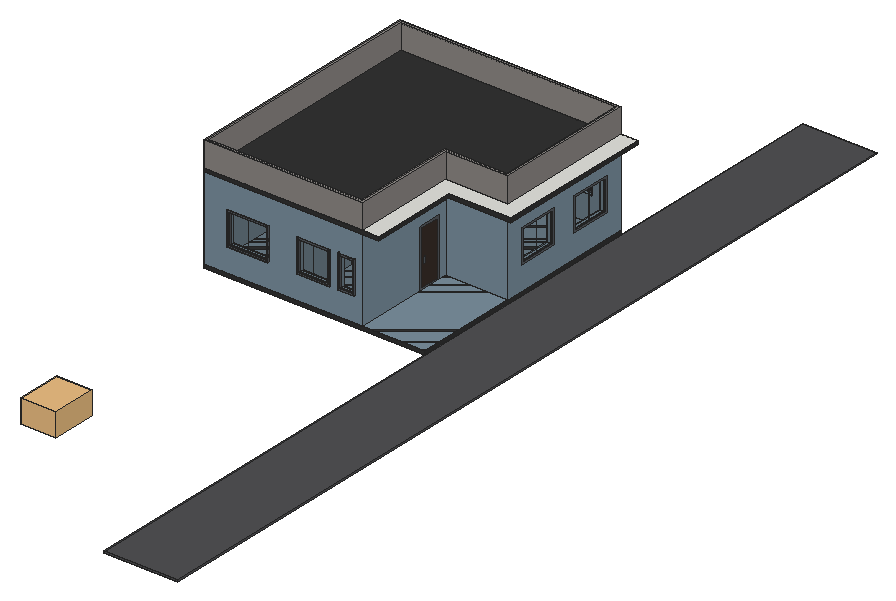
# SketchUp Ruby script. Lengths in inches.
U = 1.inch
M = Sketchup.active_model
def pt(a) = Geom::Point3d.new(a.map { |v| v * U })
def face(e, loops, mat)
  f = e.add_face(loops[0].map { |a| pt(a) })
  loops[1..].each { |l| e.add_face(l.map { |a| pt(a) }).erase! }
  f.material = f.back_material = mat if mat
  f
end
# faces: each face lists its corners as indices into pts; further lists are holes
def faces(e, pts, list, mat = nil) = list.each { |f| face(e, (f[0].is_a?(Array) ? f : [f]).map { |l| l.map { |i| pts[i] } }, mat) }
# xy, xz, yz: faces in a plane at the given z, y or x. An outline is a flat list of corners, or four numbers for a rectangle; further outlines are holes
def ring(l) = l.size == 4 ? [[l[0], l[1]], [l[2], l[1]], [l[2], l[3]], [l[0], l[3]]] : l.each_slice(2).to_a
def flat(e, list, mat, &to3) = list.each { |f| face(e, (f[0].is_a?(Array) ? f : [f]).map { |l| ring(l).map { |u, v| to3.(u, v) } }, mat) }
def xy(e, z, list, mat = nil) = flat(e, list, mat) { |x, y| [x, y, z] }
def xz(e, y, list, mat = nil) = flat(e, list, mat) { |x, z| [x, y, z] }
def yz(e, x, list, mat = nil) = flat(e, list, mat) { |y, z| [x, y, z] }
def lines(e, pts, list) = list.each { |a, b| e.add_line(pt(pts[a]), pt(pts[b])) }
# prism: a flat outline (further loops are holes) pulled along v
def prism(e, loops, v, mat = nil)
  f = face(e, loops, mat); d = Geom::Vector3d.new(v.map { |x| x * U })
  f.pushpull(f.normal.samedirection?(d) ? d.length : -d.length)
end
def box(e, o, s, mat = nil) = prism(e, [[o, [o[0] + s[0], o[1], o[2]], [o[0] + s[0], o[1] + s[1], o[2]], [o[0], o[1] + s[1], o[2]]]], [0, 0, s[2]], mat)
def at(x, y, z, deg = 0) = Geom::Transformation.translation(pt([x, y, z])) * Geom::Transformation.rotation(ORIGIN, Z_AXIS, deg.degrees)
def axes(o, x, y, z) = Geom::Transformation.new([*x, 0, *y, 0, *z, 0, *pt(o).to_a, 1])
def part(name) = M.definitions.add(name)
# library, detail: a bought-in or finely detailed component or shape, given as its bounding box
def library(name, o, s) = part(name).tap { |d| box(d.entities, o, s) }
def detail(e, o, s) = box(e.add_group.entities, o, s)
def put(e, d, t, mat = nil) = e.add_instance(d, t).tap { |i| i.material = mat if mat }
def group(e, t, mat = nil) = e.add_group.tap { |g| g.transformation = t; g.material = mat if mat }.entities
root = M.entities
M.materials.add("Asphalt A01 100cm").color = [81, 81, 83]
M.materials.add("Glass Smoked Distorted 001").color = [38, 38, 38]
M.materials["Glass Smoked Distorted 001"].alpha = 0.1
M.materials.add("Metal Sandblasted Black 200cm").color = [86, 90, 95]
M.materials.add("Two Color Maple Panels 300cm").color = [56, 46, 41]
M.materials.add("Venetian Plaster Black 300cm").color = [50, 50, 50]
M.materials.add("Wall Paint Dusk Blue Semigloss 300cm").color = [122, 143, 157]
M.materials.add("Wall Paint Poised Taupe Satin 300cm").color = [140, 135, 132]
c1 = library("Dome Light",[-12,-12,0],[24,24,12])
c2 = part("Group\#18")
box(c2.entities,[0,0,0],[28,0.31,44])
c3 = part("Group\#20")
box(c3.entities,[0,0,0],[22,0.31,44])
c4 = part("Group\#24")
box(c4.entities,[-0.31,0,0],[0.31,28,44])
c5 = part("Group\#26")
box(c5.entities,[-0.31,0,0],[0.31,28,44])
c6 = part("Group\#28")
box(c6.entities,[0,-0.31,0],[28,0.31,44])
c7 = part("Group\#30")
box(c7.entities,[0,-0.31,0],[28,0.31,44])
c8 = part("Group\#32")
box(c8.entities,[-0.31,0,0],[0.31,20,2])
c9 = part("Group\#34")
box(c9.entities,[-0.31,0,0],[0.31,20,2])
xy(root,137.15,[[234.81,586.875,258.81,586.875,258.81,714.875,349.81,714.875,349.81,946.875,325.81,946.875,325.81,738.875,234.81,738.875]])
put(root,c1,axes([-34.36,362.21,-107.93],[2.18,0,0],[0,2.76,0],[0,0,2.81]))
g1 = group(root,at(1.81,586.875,11.15))
xy(g1,0,[[233,0,324,0,324,152,233,152,233,140,228.5,140,228.5,161,315,161,315,351,192,351,192,279,187.5,279,187.5,351,61.5,351,61.5,339,57,339,57,351,9,351,9,267,57,267,57,303,61.5,303,61.5,231,187.5,231,187.5,243,192,243,192,226.5,61.5,226.5,61.5,154.5,133.5,154.5,133.5,138,129,138,129,150,51,150,51,154.5,57,154.5,57,226.5,9,226.5,9,154.5,15,154.5,15,150,9,150,9,9,129,9,129,102,133.5,102,133.5,9,228.5,9,228.5,87,169.5,87,169.5,91.5,228.5,91.5,228.5,104,233,104],[9,231,57,262.5]],"Wall Paint Dusk Blue Semigloss 300cm")
xy(g1,36,[[36,0,96,9],[137.6875,0,185.6875,9],[197.6875,0,221.6875,9],[315,175.5625,324,235.5625],[315,271.5625,324,331.5625],
  [93.4375,351,153.4375,360],[228,351,288,360]],"Wall Paint Dusk Blue Semigloss 300cm")
xy(g1,60,[[0,185.3125,9,209.3125],[0,292.25,9,316.25]],"Wall Paint Dusk Blue Semigloss 300cm")
xy(g1,84,[[36,0,96,9],[137.6875,0,185.6875,9],[197.6875,0,221.6875,9],[133.5,87,169.5,91.5],[129,102,133.5,138],
  [228.5,104,233,140],[15,150,51,154.5],[315,175.5625,324,235.5625],[0,185.3125,9,209.3125],[187.5,243,192,279],
  [315,271.5625,324,331.5625],[0,292.25,9,316.25],[57,303,61.5,339],[93.4375,351,153.4375,360],[228,351,288,360]],"Wall Paint Dusk Blue Semigloss 300cm")
xy(g1,120,[[[0,0,233,0,233,152,324,152,324,360,0,360],[133.5,91.5,133.5,154.5,61.5,154.5,61.5,226.5,192,226.5,192,351,315,351,315,161,228.5,161,228.5,91.5],[9,9,129,150],[61.5,231,187.5,351],[133.5,9,228.5,87],[9,154.5,9,262.5,57,262.5,57,231,9,231,9,226.5,57,226.5,57,154.5],[9,267,57,351]]],"Wall Paint Dusk Blue Semigloss 300cm")
xz(g1,0,[[[0,0,233,120],[36,36,96,84],[137.6875,36,185.6875,84],[197.6875,36,221.6875,84]]],"Wall Paint Dusk Blue Semigloss 300cm")
xz(g1,9,[[[9,0,129,120],[36,36,96,84]],[[133.5,0,228.5,120],[137.6875,36,185.6875,84],[197.6875,36,221.6875,84]]],"Wall Paint Dusk Blue Semigloss 300cm")
xz(g1,87,[[169.5,0,228.5,0,228.5,120,133.5,120,133.5,84,169.5,84]],"Wall Paint Dusk Blue Semigloss 300cm")
xz(g1,91.5,[[169.5,0,169.5,84,133.5,84,133.5,120,228.5,120,228.5,0]],"Wall Paint Dusk Blue Semigloss 300cm")
xz(g1,102,[[129,0,133.5,84]],"Wall Paint Dusk Blue Semigloss 300cm")
xz(g1,104,[[228.5,0,233,84]],"Wall Paint Dusk Blue Semigloss 300cm")
xz(g1,138,[[129,0,133.5,84]],"Wall Paint Dusk Blue Semigloss 300cm")
xz(g1,140,[[228.5,0,233,84]],"Wall Paint Dusk Blue Semigloss 300cm")
xz(g1,150,[[9,0,15,0,15,84,51,84,51,0,129,0,129,120,9,120]],"Wall Paint Dusk Blue Semigloss 300cm")
xz(g1,152,[[233,0,324,120]],"Wall Paint Dusk Blue Semigloss 300cm")
xz(g1,154.5,[[9,0,9,120,57,120,57,0,51,0,51,84,15,84,15,0],[61.5,0,133.5,120]],"Wall Paint Dusk Blue Semigloss 300cm")
xz(g1,161,[[228.5,0,315,120]],"Wall Paint Dusk Blue Semigloss 300cm")
xz(g1,175.5625,[[315,36,324,84]],"Wall Paint Dusk Blue Semigloss 300cm")
xz(g1,185.3125,[[0,60,9,84]],"Wall Paint Dusk Blue Semigloss 300cm")
xz(g1,209.3125,[[0,60,9,84]],"Wall Paint Dusk Blue Semigloss 300cm")
xz(g1,226.5,[[9,0,57,120],[61.5,0,192,120]],"Wall Paint Dusk Blue Semigloss 300cm")
xz(g1,231,[[9,0,57,120],[61.5,0,187.5,120]],"Wall Paint Dusk Blue Semigloss 300cm")
xz(g1,235.5625,[[315,36,324,84]],"Wall Paint Dusk Blue Semigloss 300cm")
xz(g1,243,[[187.5,0,192,84]],"Wall Paint Dusk Blue Semigloss 300cm")
xz(g1,262.5,[[9,0,57,120]],"Wall Paint Dusk Blue Semigloss 300cm")
xz(g1,267,[[9,0,57,120]],"Wall Paint Dusk Blue Semigloss 300cm")
xz(g1,271.5625,[[315,36,324,84]],"Wall Paint Dusk Blue Semigloss 300cm")
xz(g1,279,[[187.5,0,192,84]],"Wall Paint Dusk Blue Semigloss 300cm")
xz(g1,292.25,[[0,60,9,84]],"Wall Paint Dusk Blue Semigloss 300cm")
xz(g1,303,[[57,0,61.5,84]],"Wall Paint Dusk Blue Semigloss 300cm")
xz(g1,316.25,[[0,60,9,84]],"Wall Paint Dusk Blue Semigloss 300cm")
xz(g1,331.5625,[[315,36,324,84]],"Wall Paint Dusk Blue Semigloss 300cm")
xz(g1,339,[[57,0,61.5,84]],"Wall Paint Dusk Blue Semigloss 300cm")
xz(g1,351,[[9,0,57,120],[[61.5,0,187.5,120],[93.4375,36,153.4375,84]],[[192,0,315,120],[228,36,288,84]]],"Wall Paint Dusk Blue Semigloss 300cm")
xz(g1,360,[[[0,0,324,120],[228,36,288,84],[93.4375,36,153.4375,84]]],"Wall Paint Dusk Blue Semigloss 300cm")
yz(g1,0,[[[0,0,360,120],[292.25,60,316.25,84],[185.3125,60,209.3125,84]]],"Wall Paint Dusk Blue Semigloss 300cm")
yz(g1,9,[[9,0,150,120],[[154.5,0,226.5,120],[185.3125,60,209.3125,84]],[226.5,0,231,120],[231,0,262.5,120],[[267,0,351,120],[292.25,60,316.25,84]]],"Wall Paint Dusk Blue Semigloss 300cm")
yz(g1,15,[[150,0,154.5,84]],"Wall Paint Dusk Blue Semigloss 300cm")
yz(g1,36,[[0,36,9,84]],"Wall Paint Dusk Blue Semigloss 300cm")
yz(g1,51,[[150,0,154.5,84]],"Wall Paint Dusk Blue Semigloss 300cm")
yz(g1,57,[[154.5,0,226.5,120],[231,0,262.5,120],[267,0,267,120,351,120,351,0,339,0,339,84,303,84,303,0]],"Wall Paint Dusk Blue Semigloss 300cm")
yz(g1,61.5,[[154.5,0,226.5,120],[231,0,303,0,303,84,339,84,339,0,351,0,351,120,231,120]],"Wall Paint Dusk Blue Semigloss 300cm")
yz(g1,93.4375,[[351,36,360,84]],"Wall Paint Dusk Blue Semigloss 300cm")
yz(g1,96,[[0,36,9,84]],"Wall Paint Dusk Blue Semigloss 300cm")
yz(g1,129,[[9,0,9,120,150,120,150,0,138,0,138,84,102,84,102,0]],"Wall Paint Dusk Blue Semigloss 300cm")
yz(g1,133.5,[[9,0,102,0,102,84,138,84,138,0,154.5,0,154.5,120,91.5,120,91.5,84,87,84,87,120,9,120]],"Wall Paint Dusk Blue Semigloss 300cm")
yz(g1,137.6875,[[0,36,9,84]],"Wall Paint Dusk Blue Semigloss 300cm")
yz(g1,153.4375,[[351,36,360,84]],"Wall Paint Dusk Blue Semigloss 300cm")
yz(g1,169.5,[[87,0,91.5,84]],"Wall Paint Dusk Blue Semigloss 300cm")
yz(g1,185.6875,[[0,36,9,84]],"Wall Paint Dusk Blue Semigloss 300cm")
yz(g1,187.5,[[231,0,231,120,351,120,351,0,279,0,279,84,243,84,243,0]],"Wall Paint Dusk Blue Semigloss 300cm")
yz(g1,192,[[226.5,0,243,0,243,84,279,84,279,0,351,0,351,120,226.5,120]],"Wall Paint Dusk Blue Semigloss 300cm")
yz(g1,197.6875,[[0,36,9,84]],"Wall Paint Dusk Blue Semigloss 300cm")
yz(g1,221.6875,[[0,36,9,84]],"Wall Paint Dusk Blue Semigloss 300cm")
yz(g1,228,[[351,36,360,84]],"Wall Paint Dusk Blue Semigloss 300cm")
yz(g1,228.5,[[9,0,87,120],[91.5,0,91.5,120,161,120,161,0,140,0,140,84,104,84,104,0]],"Wall Paint Dusk Blue Semigloss 300cm")
yz(g1,233,[[0,0,104,0,104,84,140,84,140,0,152,0,152,120,0,120]],"Wall Paint Dusk Blue Semigloss 300cm")
yz(g1,288,[[351,36,360,84]],"Wall Paint Dusk Blue Semigloss 300cm")
yz(g1,315,[[[161,0,351,120],[175.5625,36,235.5625,84],[271.5625,36,331.5625,84]]],"Wall Paint Dusk Blue Semigloss 300cm")
yz(g1,324,[[[152,0,360,120],[175.5625,36,235.5625,84],[271.5625,36,331.5625,84]]],"Wall Paint Dusk Blue Semigloss 300cm")
g2 = group(g1,at(233,104,0))
prism(g2,[[[0,36,0],[0,36,84],[0,0,84],[0,0,0]],[[0,2,82],[0,34,82],[0,34,2],[0,2,2]]],[-2.5,0,0],"Metal Sandblasted Black 200cm")
g3 = group(g2,at(0,2,2))
xy(g3,0,[[-0.71,0,0,32]])
xy(g3,80,[[-0.71,0,0,32]])
xz(g3,0,[[-0.71,0,0,80]])
xz(g3,32,[[-0.71,0,0,80]])
yz(g3,-0.71,[[0,0,32,80]])
yz(g3,0,[[0,0,32,80]],"Two Color Maple Panels 300cm")
g4 = group(g3,at(0,6,32),"Metal Sandblasted Black 200cm")
box(g4,[0,0,0],[0.5,1.5,8])
g5 = group(g1,at(133.5,102,0))
prism(g5,[[[0,36,0],[0,36,84],[0,0,84],[0,0,0]],[[0,34,82],[0,34,2],[0,2,2],[0,2,82]]],[-2.5,0,0])
g6 = group(g5,at(0,2,2))
box(g6,[-0.71,0,0],[0.71,32,80])
g7 = group(g6,at(0,6,32))
box(g7,[0,0,0],[0.5,1.5,8])
g8 = group(g1,at(15,150,0))
prism(g8,[[[36,0,0],[36,0,84],[0,0,84],[0,0,0]],[[2,0,2],[2,0,82],[34,0,82],[34,0,2]]],[0,2.5,0])
g9 = group(g8,at(2,0,2))
box(g9,[0,0,0],[32,0.71,80])
g10 = group(g9,at(6,0,32))
box(g10,[0,-0.5,0],[1.5,0.5,8])
g11 = group(g1,at(192,243,0))
prism(g11,[[[0,36,0],[0,36,84],[0,0,84],[0,0,0]],[[0,2,82],[0,34,82],[0,34,2],[0,2,2]]],[-2.5,0,0])
g12 = group(g11,at(0,2,2))
yz(g12,0,[[0,0,32,80]])
g13 = group(g12,at(0,6,32))
box(g13,[0,0,0],[0.5,1.5,8])
g14 = group(g1,at(61.5,303,0))
prism(g14,[[[0,36,0],[0,36,84],[0,0,84],[0,0,0]],[[0,34,2],[0,2,2],[0,2,82],[0,34,82]]],[-2.5,0,0])
g15 = group(g14,at(0,2,2))
box(g15,[-0.71,0,0],[0.71,32,80])
g16 = group(g15,at(0,6,32))
box(g16,[0,0,0],[0.5,1.5,8])
g17 = group(g1,at(36,0,36))
prism(g17,[[[0,-1.5,0],[60,-1.5,0],[60,-1.5,48],[0,-1.5,48]],[[58,-1.5,46],[58,-1.5,2],[2,-1.5,2],[2,-1.5,46]]],[0,3,0],"Metal Sandblasted Black 200cm")
put(g17,c2,at(2,-0.125,2),"Glass Smoked Distorted 001")
put(g17,c2,at(30,-0.44,2),"Glass Smoked Distorted 001")
g18 = group(g1,at(137.6875,0,36))
prism(g18,[[[48,1.5,48],[48,1.5,0],[0,1.5,0],[0,1.5,48]],[[46,1.5,2],[46,1.5,46],[2,1.5,46],[2,1.5,2]]],[0,-3,0],"Metal Sandblasted Black 200cm")
put(g18,c3,at(2,0.0625,2),"Glass Smoked Distorted 001")
put(g18,c3,at(24,-0.25,2),"Glass Smoked Distorted 001")
g19 = group(g1,at(197.6875,0,36))
prism(g19,[[[24,-1.5,0],[24,-1.5,48],[0,-1.5,48],[0,-1.5,0]],[[2,-1.5,2],[2,-1.5,46],[22,-1.5,46],[22,-1.5,2]]],[0,3,0],"Metal Sandblasted Black 200cm")
g20 = group(g19,at(2,-0.125,2))
box(g20,[0,0,0],[20,0.31,44],"Glass Smoked Distorted 001")
g21 = group(g1,at(324,175.5625,36))
prism(g21,[[[1.5,60,0],[1.5,60,48],[1.5,0,48],[1.5,0,0]],[[1.5,58,2],[1.5,2,2],[1.5,2,46],[1.5,58,46]]],[-3,0,0],"Metal Sandblasted Black 200cm")
put(g21,c4,at(-0.0625,2,2),"Glass Smoked Distorted 001")
put(g21,c4,at(0.25,30,2),"Glass Smoked Distorted 001")
g22 = group(g1,at(324,271.5625,36))
prism(g22,[[[1.5,0,0],[1.5,60,0],[1.5,60,48],[1.5,0,48]],[[1.5,58,46],[1.5,58,2],[1.5,2,2],[1.5,2,46]]],[-3,0,0],"Metal Sandblasted Black 200cm")
put(g22,c5,at(0.1875,2,2),"Glass Smoked Distorted 001")
put(g22,c5,at(0.5,30,2),"Glass Smoked Distorted 001")
g23 = group(g1,at(228,360,36))
prism(g23,[[[60,1.5,0],[0,1.5,0],[0,1.5,48],[60,1.5,48]],[[58,1.5,46],[2,1.5,46],[2,1.5,2],[58,1.5,2]]],[0,-4,0],"Metal Sandblasted Black 200cm")
put(g23,c6,at(30,-0.9375,2),"Glass Smoked Distorted 001")
put(g23,c6,at(2,-0.62,2),"Glass Smoked Distorted 001")
g24 = group(g1,at(93.4375,360,36))
prism(g24,[[[60,1.5,0],[0,1.5,0],[0,1.5,48],[60,1.5,48]],[[2,1.5,2],[58,1.5,2],[58,1.5,46],[2,1.5,46]]],[0,-3,0],"Metal Sandblasted Black 200cm")
put(g24,c7,at(30,-0.125,2),"Glass Smoked Distorted 001")
put(g24,c7,at(2,0.19,2),"Glass Smoked Distorted 001")
g25 = group(g1,at(0,292.25,60))
prism(g25,[[[-1.5,24,0],[-1.5,0,0],[-1.5,0,24],[-1.5,24,24]],[[-1.5,22,22],[-1.5,2,22],[-1.5,2,2],[-1.5,22,2]]],[3,0,0],"Metal Sandblasted Black 200cm")
put(g25,c8,at(-1.5,2,20),"Glass Smoked Distorted 001")
put(g25,c8,at(-1.5,2,17),"Glass Smoked Distorted 001")
put(g25,c8,at(-1.5,2,14),"Glass Smoked Distorted 001")
put(g25,c8,at(-1.5,2,11),"Glass Smoked Distorted 001")
put(g25,c8,at(-1.5,2,8),"Glass Smoked Distorted 001")
put(g25,c8,at(-1.5,2,5),"Glass Smoked Distorted 001")
put(g25,c8,at(-1.5,2,2),"Glass Smoked Distorted 001")
g26 = group(g1,at(0,185.3125,60))
prism(g26,[[[-1.5,24,0],[-1.5,0,0],[-1.5,0,24],[-1.5,24,24]],[[-1.5,22,22],[-1.5,2,22],[-1.5,2,2],[-1.5,22,2]]],[3,0,0],"Metal Sandblasted Black 200cm")
put(g26,c9,at(-1.5,2,20),"Glass Smoked Distorted 001")
put(g26,c9,at(-1.5,2,17),"Glass Smoked Distorted 001")
put(g26,c9,at(-1.5,2,14),"Glass Smoked Distorted 001")
put(g26,c9,at(-1.5,2,11),"Glass Smoked Distorted 001")
put(g26,c9,at(-1.5,2,8),"Glass Smoked Distorted 001")
put(g26,c9,at(-1.5,2,5),"Glass Smoked Distorted 001")
put(g26,c9,at(-1.5,2,2),"Glass Smoked Distorted 001")
g27 = group(root,at(1.81,586.875,131.15))
prism(g27,[[[257,128,0],[257,0,0],[0,0,0],[0,360,0],[348,360,0],[348,128,0]]],[0,0,6],"Venetian Plaster Black 300cm")
g28 = group(g27,at(0,0,6))
prism(g28,[[[233,152,0],[233,0,0],[0,0,0],[0,360,0],[324,360,0],[324,152,0]],[[319.5,156.5,0],[319.5,355.5,0],[4.5,355.5,0],[4.5,4.5,0],[228.5,4.5,0],[228.5,156.5,0]]],[0,0,36],"Wall Paint Poised Taupe Satin 300cm")
g29 = group(root,at(1.81,586.875,11.15))
box(g29,[0,0,-6],[324,360,6],"Venetian Plaster Black 300cm")
g30 = group(root,at(325.81,586.875,5.15),"Asphalt A01 100cm")
box(g30,[0,-586.875,-2],[108.3125,1278.875,2],"Asphalt A01 100cm")
